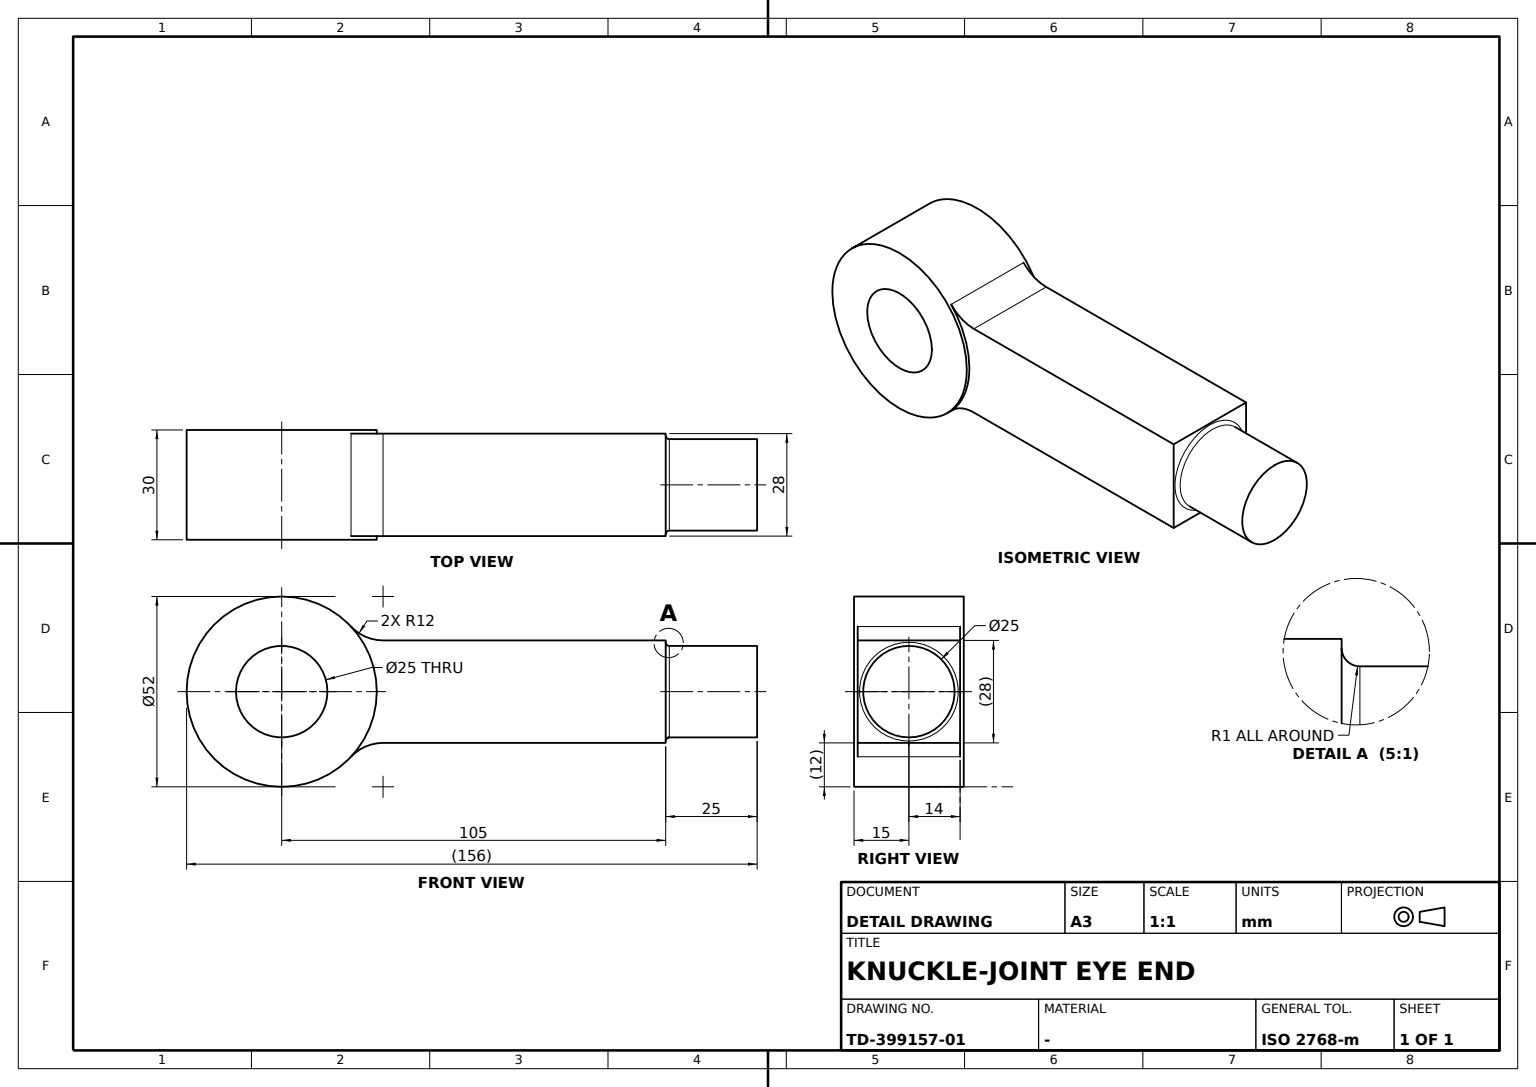
ISO-10303-21;
HEADER;
FILE_DESCRIPTION((''),'2;1');
FILE_NAME('','',(''),(''),'','','');
FILE_SCHEMA(('AUTOMOTIVE_DESIGN'));
ENDSEC;
DATA;
#1=APPLICATION_CONTEXT('');
#2=PRODUCT_CONTEXT('',#1,'mechanical');
#3=PRODUCT('','','',(#2));
#4=PRODUCT_DEFINITION_FORMATION('','',#3);
#5=PRODUCT_DEFINITION_CONTEXT('',#1,'design');
#6=PRODUCT_DEFINITION('','',#4,#5);
#7=PRODUCT_DEFINITION_SHAPE('','',#6);
#8=(LENGTH_UNIT()NAMED_UNIT(*)SI_UNIT(.MILLI.,.METRE.));
#9=(NAMED_UNIT(*)PLANE_ANGLE_UNIT()SI_UNIT($,.RADIAN.));
#10=(NAMED_UNIT(*)SI_UNIT($,.STERADIAN.)SOLID_ANGLE_UNIT());
#11=UNCERTAINTY_MEASURE_WITH_UNIT(LENGTH_MEASURE(1.E-05),#8,'distance_accuracy_value','');
#12=(GEOMETRIC_REPRESENTATION_CONTEXT(3)GLOBAL_UNCERTAINTY_ASSIGNED_CONTEXT((#11))GLOBAL_UNIT_ASSIGNED_CONTEXT((#8,#9,#10))REPRESENTATION_CONTEXT('',''));
#13=CARTESIAN_POINT('',(0.,-26.,-15.));
#14=VERTEX_POINT('',#13);
#15=CARTESIAN_POINT('',(0.,26.,-15.));
#16=VERTEX_POINT('',#15);
#17=CARTESIAN_POINT('',(0.,0.,-15.));
#18=DIRECTION('',(0.,0.,1.));
#19=DIRECTION('',(0.,-1.,0.));
#20=AXIS2_PLACEMENT_3D('',#17,#18,#19);
#21=CIRCLE('',#20,26.);
#22=EDGE_CURVE('',#14,#16,#21,.T.);
#23=ORIENTED_EDGE('',*,*,#22,.F.);
#24=EDGE_CURVE('',#16,#14,#21,.T.);
#25=ORIENTED_EDGE('',*,*,#24,.F.);
#26=EDGE_LOOP('',(#23,#25));
#27=FACE_OUTER_BOUND('',#26,.T.);
#28=CARTESIAN_POINT('',(0.,12.5,-15.));
#29=VERTEX_POINT('',#28);
#30=CARTESIAN_POINT('',(0.,-12.5,-15.));
#31=VERTEX_POINT('',#30);
#32=CIRCLE('',#20,12.5);
#33=EDGE_CURVE('',#29,#31,#32,.T.);
#34=ORIENTED_EDGE('',*,*,#33,.T.);
#35=EDGE_CURVE('',#31,#29,#32,.T.);
#36=ORIENTED_EDGE('',*,*,#35,.T.);
#37=EDGE_LOOP('',(#34,#36));
#38=FACE_BOUND('',#37,.T.);
#39=PLANE('',#20);
#40=ADVANCED_FACE('',(#27,#38),#39,.F.);
#41=CARTESIAN_POINT('',(0.,-12.5,14.));
#42=VERTEX_POINT('',#41);
#43=CARTESIAN_POINT('',(0.,-12.5,-14.));
#44=VERTEX_POINT('',#43);
#45=CARTESIAN_POINT('',(0.,-12.5,6.84));
#46=DIRECTION('',(0.,0.,-1.));
#47=VECTOR('',#46,1000.);
#48=LINE('',#45,#47);
#49=EDGE_CURVE('',#42,#44,#48,.T.);
#50=ORIENTED_EDGE('',*,*,#49,.F.);
#51=CARTESIAN_POINT('',(0.,12.5,14.));
#52=VERTEX_POINT('',#51);
#53=CARTESIAN_POINT('',(0.,0.,14.));
#54=DIRECTION('',(0.,1.,0.));
#55=AXIS2_PLACEMENT_3D('',#53,#18,#54);
#56=CIRCLE('',#55,12.5);
#57=EDGE_CURVE('',#42,#52,#56,.T.);
#58=ORIENTED_EDGE('',*,*,#57,.T.);
#59=CARTESIAN_POINT('',(0.,12.5,-14.));
#60=VERTEX_POINT('',#59);
#61=CARTESIAN_POINT('',(0.,12.5,6.84));
#62=LINE('',#61,#47);
#63=EDGE_CURVE('',#52,#60,#62,.T.);
#64=ORIENTED_EDGE('',*,*,#63,.T.);
#65=CARTESIAN_POINT('',(0.,0.,-14.));
#66=AXIS2_PLACEMENT_3D('',#65,#18,#54);
#67=CIRCLE('',#66,12.5);
#68=EDGE_CURVE('',#44,#60,#67,.T.);
#69=ORIENTED_EDGE('',*,*,#68,.F.);
#70=EDGE_LOOP('',(#50,#58,#64,#69));
#71=FACE_OUTER_BOUND('',#70,.T.);
#72=CARTESIAN_POINT('',(0.,0.,6.84));
#73=AXIS2_PLACEMENT_3D('',#72,#46,#54);
#74=CYLINDRICAL_SURFACE('',#73,12.5);
#75=ADVANCED_FACE('',(#71),#74,.F.);
#76=CARTESIAN_POINT('',(0.,12.5,15.));
#77=VERTEX_POINT('',#76);
#78=CARTESIAN_POINT('',(0.,-12.5,15.));
#79=VERTEX_POINT('',#78);
#80=CARTESIAN_POINT('',(0.,0.,15.));
#81=AXIS2_PLACEMENT_3D('',#80,#18,#19);
#82=CIRCLE('',#81,12.5);
#83=EDGE_CURVE('',#77,#79,#82,.T.);
#84=ORIENTED_EDGE('',*,*,#83,.F.);
#85=EDGE_CURVE('',#79,#77,#82,.T.);
#86=ORIENTED_EDGE('',*,*,#85,.F.);
#87=EDGE_LOOP('',(#84,#86));
#88=FACE_BOUND('',#87,.T.);
#89=CARTESIAN_POINT('',(0.,26.,15.));
#90=VERTEX_POINT('',#89);
#91=CARTESIAN_POINT('',(0.,-26.,15.));
#92=VERTEX_POINT('',#91);
#93=CIRCLE('',#81,26.);
#94=EDGE_CURVE('',#90,#92,#93,.T.);
#95=ORIENTED_EDGE('',*,*,#94,.T.);
#96=EDGE_CURVE('',#92,#90,#93,.T.);
#97=ORIENTED_EDGE('',*,*,#96,.T.);
#98=EDGE_LOOP('',(#95,#97));
#99=FACE_OUTER_BOUND('',#98,.T.);
#100=PLANE('',#81);
#101=ADVANCED_FACE('',(#88,#99),#100,.T.);
#102=ORIENTED_EDGE('',*,*,#63,.F.);
#103=EDGE_CURVE('',#52,#42,#56,.T.);
#104=ORIENTED_EDGE('',*,*,#103,.T.);
#105=ORIENTED_EDGE('',*,*,#49,.T.);
#106=EDGE_CURVE('',#60,#44,#67,.T.);
#107=ORIENTED_EDGE('',*,*,#106,.F.);
#108=EDGE_LOOP('',(#102,#104,#105,#107));
#109=FACE_OUTER_BOUND('',#108,.T.);
#110=ADVANCED_FACE('',(#109),#74,.F.);
#111=CARTESIAN_POINT('',(12.5,106.,0.));
#112=VERTEX_POINT('',#111);
#113=CARTESIAN_POINT('',(-12.5,106.,0.));
#114=VERTEX_POINT('',#113);
#115=CARTESIAN_POINT('',(0.,106.,0.));
#116=DIRECTION('',(-1.,0.,0.));
#117=AXIS2_PLACEMENT_3D('',#115,#19,#116);
#118=CIRCLE('',#117,12.5);
#119=EDGE_CURVE('',#112,#114,#118,.T.);
#120=ORIENTED_EDGE('',*,*,#119,.F.);
#121=CARTESIAN_POINT('',(12.5,130.,0.));
#122=VERTEX_POINT('',#121);
#123=CARTESIAN_POINT('',(12.5,117.5,0.));
#124=VECTOR('',#54,1000.);
#125=LINE('',#123,#124);
#126=EDGE_CURVE('',#112,#122,#125,.T.);
#127=ORIENTED_EDGE('',*,*,#126,.T.);
#128=CARTESIAN_POINT('',(-12.5,130.,0.));
#129=VERTEX_POINT('',#128);
#130=CARTESIAN_POINT('',(0.,130.,0.));
#131=AXIS2_PLACEMENT_3D('',#130,#54,#116);
#132=CIRCLE('',#131,12.5);
#133=EDGE_CURVE('',#129,#122,#132,.T.);
#134=ORIENTED_EDGE('',*,*,#133,.F.);
#135=CARTESIAN_POINT('',(-12.5,117.5,0.));
#136=LINE('',#135,#124);
#137=EDGE_CURVE('',#114,#129,#136,.T.);
#138=ORIENTED_EDGE('',*,*,#137,.F.);
#139=EDGE_LOOP('',(#120,#127,#134,#138));
#140=FACE_OUTER_BOUND('',#139,.T.);
#141=CARTESIAN_POINT('',(0.,117.5,0.));
#142=AXIS2_PLACEMENT_3D('',#141,#19,#116);
#143=CYLINDRICAL_SURFACE('',#142,12.5);
#144=ADVANCED_FACE('',(#140),#143,.T.);
#145=CARTESIAN_POINT('',(0.,-12.5,0.));
#146=VECTOR('',#18,1000.);
#147=LINE('',#145,#146);
#148=EDGE_CURVE('',#42,#79,#147,.T.);
#149=ORIENTED_EDGE('',*,*,#148,.F.);
#150=ORIENTED_EDGE('',*,*,#103,.F.);
#151=CARTESIAN_POINT('',(0.,12.5,0.));
#152=LINE('',#151,#146);
#153=EDGE_CURVE('',#52,#77,#152,.T.);
#154=ORIENTED_EDGE('',*,*,#153,.T.);
#155=ORIENTED_EDGE('',*,*,#83,.T.);
#156=EDGE_LOOP('',(#149,#150,#154,#155));
#157=FACE_OUTER_BOUND('',#156,.T.);
#158=CARTESIAN_POINT('',(0.,0.,0.));
#159=AXIS2_PLACEMENT_3D('',#158,#46,#19);
#160=CYLINDRICAL_SURFACE('',#159,12.5);
#161=ADVANCED_FACE('',(#157),#160,.F.);
#162=EDGE_CURVE('',#31,#44,#147,.T.);
#163=ORIENTED_EDGE('',*,*,#162,.F.);
#164=ORIENTED_EDGE('',*,*,#33,.F.);
#165=EDGE_CURVE('',#29,#60,#152,.T.);
#166=ORIENTED_EDGE('',*,*,#165,.T.);
#167=ORIENTED_EDGE('',*,*,#106,.T.);
#168=EDGE_LOOP('',(#163,#164,#166,#167));
#169=FACE_OUTER_BOUND('',#168,.T.);
#170=ADVANCED_FACE('',(#169),#160,.F.);
#171=ORIENTED_EDGE('',*,*,#137,.T.);
#172=EDGE_CURVE('',#122,#129,#132,.T.);
#173=ORIENTED_EDGE('',*,*,#172,.F.);
#174=ORIENTED_EDGE('',*,*,#126,.F.);
#175=EDGE_CURVE('',#114,#112,#118,.T.);
#176=ORIENTED_EDGE('',*,*,#175,.F.);
#177=EDGE_LOOP('',(#171,#173,#174,#176));
#178=FACE_OUTER_BOUND('',#177,.T.);
#179=ADVANCED_FACE('',(#178),#143,.T.);
#180=CARTESIAN_POINT('',(0.,26.,-14.));
#181=VERTEX_POINT('',#180);
#182=CARTESIAN_POINT('',(0.,26.,0.));
#183=LINE('',#182,#146);
#184=EDGE_CURVE('',#16,#181,#183,.T.);
#185=ORIENTED_EDGE('',*,*,#184,.F.);
#186=ORIENTED_EDGE('',*,*,#24,.T.);
#187=CARTESIAN_POINT('',(0.,-26.,0.));
#188=LINE('',#187,#146);
#189=EDGE_CURVE('',#14,#92,#188,.T.);
#190=ORIENTED_EDGE('',*,*,#189,.T.);
#191=ORIENTED_EDGE('',*,*,#94,.F.);
#192=CARTESIAN_POINT('',(0.,26.,14.));
#193=VERTEX_POINT('',#192);
#194=EDGE_CURVE('',#193,#90,#183,.T.);
#195=ORIENTED_EDGE('',*,*,#194,.F.);
#196=CARTESIAN_POINT('',(-17.789474,18.961398,14.));
#197=VERTEX_POINT('',#196);
#198=CIRCLE('',#55,26.);
#199=EDGE_CURVE('',#193,#197,#198,.T.);
#200=ORIENTED_EDGE('',*,*,#199,.T.);
#201=CARTESIAN_POINT('',(-17.789474,18.961398,-14.));
#202=VERTEX_POINT('',#201);
#203=CARTESIAN_POINT('',(-17.789474,18.961398,0.));
#204=LINE('',#203,#146);
#205=EDGE_CURVE('',#202,#197,#204,.T.);
#206=ORIENTED_EDGE('',*,*,#205,.F.);
#207=CIRCLE('',#66,26.);
#208=EDGE_CURVE('',#181,#202,#207,.T.);
#209=ORIENTED_EDGE('',*,*,#208,.F.);
#210=EDGE_LOOP('',(#185,#186,#190,#191,#195,#200,#206,#209));
#211=FACE_OUTER_BOUND('',#210,.T.);
#212=CYLINDRICAL_SURFACE('',#159,26.);
#213=ADVANCED_FACE('',(#211),#212,.T.);
#214=ORIENTED_EDGE('',*,*,#165,.F.);
#215=ORIENTED_EDGE('',*,*,#35,.F.);
#216=ORIENTED_EDGE('',*,*,#162,.T.);
#217=ORIENTED_EDGE('',*,*,#68,.T.);
#218=EDGE_LOOP('',(#214,#215,#216,#217));
#219=FACE_OUTER_BOUND('',#218,.T.);
#220=ADVANCED_FACE('',(#219),#160,.F.);
#221=ORIENTED_EDGE('',*,*,#199,.F.);
#222=CARTESIAN_POINT('',(17.789474,18.961398,14.));
#223=VERTEX_POINT('',#222);
#224=EDGE_CURVE('',#223,#193,#198,.T.);
#225=ORIENTED_EDGE('',*,*,#224,.F.);
#226=CARTESIAN_POINT('',(14.,27.712813,14.));
#227=VERTEX_POINT('',#226);
#228=CARTESIAN_POINT('',(26.,27.712813,14.));
#229=AXIS2_PLACEMENT_3D('',#228,#46,#54);
#230=CIRCLE('',#229,12.);
#231=EDGE_CURVE('',#223,#227,#230,.T.);
#232=ORIENTED_EDGE('',*,*,#231,.T.);
#233=CARTESIAN_POINT('',(14.,105.,14.));
#234=VERTEX_POINT('',#233);
#235=CARTESIAN_POINT('',(14.,66.356406,14.));
#236=LINE('',#235,#124);
#237=EDGE_CURVE('',#227,#234,#236,.T.);
#238=ORIENTED_EDGE('',*,*,#237,.T.);
#239=CARTESIAN_POINT('',(-14.,105.,14.));
#240=VERTEX_POINT('',#239);
#241=CARTESIAN_POINT('',(0.,105.,14.));
#242=VECTOR('',#116,1000.);
#243=LINE('',#241,#242);
#244=EDGE_CURVE('',#234,#240,#243,.T.);
#245=ORIENTED_EDGE('',*,*,#244,.T.);
#246=CARTESIAN_POINT('',(-14.,27.712813,14.));
#247=VERTEX_POINT('',#246);
#248=CARTESIAN_POINT('',(-14.,66.356406,14.));
#249=VECTOR('',#19,1000.);
#250=LINE('',#248,#249);
#251=EDGE_CURVE('',#240,#247,#250,.T.);
#252=ORIENTED_EDGE('',*,*,#251,.T.);
#253=CARTESIAN_POINT('',(-26.,27.712813,14.));
#254=AXIS2_PLACEMENT_3D('',#253,#46,#54);
#255=CIRCLE('',#254,12.);
#256=EDGE_CURVE('',#247,#197,#255,.T.);
#257=ORIENTED_EDGE('',*,*,#256,.T.);
#258=EDGE_LOOP('',(#221,#225,#232,#238,#245,#252,#257));
#259=FACE_OUTER_BOUND('',#258,.T.);
#260=PLANE('',#55);
#261=ADVANCED_FACE('',(#259),#260,.T.);
#262=CARTESIAN_POINT('',(13.5,105.,0.));
#263=VERTEX_POINT('',#262);
#264=CARTESIAN_POINT('',(-13.5,105.,0.));
#265=VERTEX_POINT('',#264);
#266=CARTESIAN_POINT('',(0.,105.,0.));
#267=DIRECTION('',(1.,0.,0.));
#268=AXIS2_PLACEMENT_3D('',#266,#19,#267);
#269=CIRCLE('',#268,13.5);
#270=EDGE_CURVE('',#263,#265,#269,.T.);
#271=ORIENTED_EDGE('',*,*,#270,.T.);
#272=EDGE_CURVE('',#265,#263,#269,.T.);
#273=ORIENTED_EDGE('',*,*,#272,.T.);
#274=EDGE_LOOP('',(#271,#273));
#275=FACE_BOUND('',#274,.T.);
#276=CARTESIAN_POINT('',(14.,105.,-14.));
#277=VERTEX_POINT('',#276);
#278=CARTESIAN_POINT('',(14.,105.,0.));
#279=LINE('',#278,#146);
#280=EDGE_CURVE('',#277,#234,#279,.T.);
#281=ORIENTED_EDGE('',*,*,#280,.F.);
#282=CARTESIAN_POINT('',(-14.,105.,-14.));
#283=VERTEX_POINT('',#282);
#284=CARTESIAN_POINT('',(0.,105.,-14.));
#285=LINE('',#284,#242);
#286=EDGE_CURVE('',#277,#283,#285,.T.);
#287=ORIENTED_EDGE('',*,*,#286,.T.);
#288=CARTESIAN_POINT('',(-14.,105.,0.));
#289=LINE('',#288,#146);
#290=EDGE_CURVE('',#283,#240,#289,.T.);
#291=ORIENTED_EDGE('',*,*,#290,.T.);
#292=ORIENTED_EDGE('',*,*,#244,.F.);
#293=EDGE_LOOP('',(#281,#287,#291,#292));
#294=FACE_OUTER_BOUND('',#293,.T.);
#295=AXIS2_PLACEMENT_3D('',#288,#19,#267);
#296=PLANE('',#295);
#297=ADVANCED_FACE('',(#275,#294),#296,.F.);
#298=ORIENTED_EDGE('',*,*,#237,.F.);
#299=CARTESIAN_POINT('',(14.,27.712813,-14.));
#300=VERTEX_POINT('',#299);
#301=CARTESIAN_POINT('',(14.,27.712813,0.));
#302=LINE('',#301,#146);
#303=EDGE_CURVE('',#300,#227,#302,.T.);
#304=ORIENTED_EDGE('',*,*,#303,.F.);
#305=CARTESIAN_POINT('',(14.,66.356406,-14.));
#306=LINE('',#305,#124);
#307=EDGE_CURVE('',#300,#277,#306,.T.);
#308=ORIENTED_EDGE('',*,*,#307,.T.);
#309=ORIENTED_EDGE('',*,*,#280,.T.);
#310=EDGE_LOOP('',(#298,#304,#308,#309));
#311=FACE_OUTER_BOUND('',#310,.T.);
#312=AXIS2_PLACEMENT_3D('',#278,#116,#19);
#313=PLANE('',#312);
#314=ADVANCED_FACE('',(#311),#313,.F.);
#315=CARTESIAN_POINT('',(17.789474,18.961398,-14.));
#316=VERTEX_POINT('',#315);
#317=CARTESIAN_POINT('',(17.789474,18.961398,0.));
#318=LINE('',#317,#146);
#319=EDGE_CURVE('',#316,#223,#318,.T.);
#320=ORIENTED_EDGE('',*,*,#319,.F.);
#321=CARTESIAN_POINT('',(26.,27.712813,-14.));
#322=AXIS2_PLACEMENT_3D('',#321,#46,#54);
#323=CIRCLE('',#322,12.);
#324=EDGE_CURVE('',#316,#300,#323,.T.);
#325=ORIENTED_EDGE('',*,*,#324,.T.);
#326=ORIENTED_EDGE('',*,*,#303,.T.);
#327=ORIENTED_EDGE('',*,*,#231,.F.);
#328=EDGE_LOOP('',(#320,#325,#326,#327));
#329=FACE_OUTER_BOUND('',#328,.T.);
#330=CARTESIAN_POINT('',(26.,27.712813,0.));
#331=AXIS2_PLACEMENT_3D('',#330,#46,#54);
#332=CYLINDRICAL_SURFACE('',#331,12.);
#333=ADVANCED_FACE('',(#329),#332,.F.);
#334=ORIENTED_EDGE('',*,*,#22,.T.);
#335=ORIENTED_EDGE('',*,*,#184,.T.);
#336=EDGE_CURVE('',#316,#181,#207,.T.);
#337=ORIENTED_EDGE('',*,*,#336,.F.);
#338=ORIENTED_EDGE('',*,*,#319,.T.);
#339=ORIENTED_EDGE('',*,*,#224,.T.);
#340=ORIENTED_EDGE('',*,*,#194,.T.);
#341=ORIENTED_EDGE('',*,*,#96,.F.);
#342=ORIENTED_EDGE('',*,*,#189,.F.);
#343=EDGE_LOOP('',(#334,#335,#337,#338,#339,#340,#341,#342));
#344=FACE_OUTER_BOUND('',#343,.T.);
#345=ADVANCED_FACE('',(#344),#212,.T.);
#346=ORIENTED_EDGE('',*,*,#119,.T.);
#347=CARTESIAN_POINT('',(-13.5,106.,0.));
#348=AXIS2_PLACEMENT_3D('',#347,#46,#116);
#349=CIRCLE('',#348,1.);
#350=EDGE_CURVE('',#114,#265,#349,.T.);
#351=ORIENTED_EDGE('',*,*,#350,.T.);
#352=ORIENTED_EDGE('',*,*,#270,.F.);
#353=CARTESIAN_POINT('',(13.5,106.,0.));
#354=DIRECTION('',(0.000000025,0.,1.));
#355=DIRECTION('',(1.,0.,-0.000000025));
#356=AXIS2_PLACEMENT_3D('',#353,#354,#355);
#357=CIRCLE('',#356,1.);
#358=EDGE_CURVE('',#112,#263,#357,.T.);
#359=ORIENTED_EDGE('',*,*,#358,.F.);
#360=EDGE_LOOP('',(#346,#351,#352,#359));
#361=FACE_OUTER_BOUND('',#360,.T.);
#362=DIRECTION('',(0.590104672,0.,-0.807326747));
#363=AXIS2_PLACEMENT_3D('',#115,#19,#362);
#364=TOROIDAL_SURFACE('',#363,13.5,1.);
#365=ADVANCED_FACE('',(#361),#364,.F.);
#366=CARTESIAN_POINT('',(-14.,27.712813,-14.));
#367=VERTEX_POINT('',#366);
#368=CARTESIAN_POINT('',(-14.,66.356406,-14.));
#369=LINE('',#368,#249);
#370=EDGE_CURVE('',#283,#367,#369,.T.);
#371=ORIENTED_EDGE('',*,*,#370,.T.);
#372=CARTESIAN_POINT('',(-14.,27.712813,0.));
#373=LINE('',#372,#146);
#374=EDGE_CURVE('',#367,#247,#373,.T.);
#375=ORIENTED_EDGE('',*,*,#374,.T.);
#376=ORIENTED_EDGE('',*,*,#251,.F.);
#377=ORIENTED_EDGE('',*,*,#290,.F.);
#378=EDGE_LOOP('',(#371,#375,#376,#377));
#379=FACE_OUTER_BOUND('',#378,.T.);
#380=AXIS2_PLACEMENT_3D('',#372,#267,#54);
#381=PLANE('',#380);
#382=ADVANCED_FACE('',(#379),#381,.F.);
#383=ORIENTED_EDGE('',*,*,#208,.T.);
#384=CARTESIAN_POINT('',(-26.,27.712813,-14.));
#385=AXIS2_PLACEMENT_3D('',#384,#46,#54);
#386=CIRCLE('',#385,12.);
#387=EDGE_CURVE('',#367,#202,#386,.T.);
#388=ORIENTED_EDGE('',*,*,#387,.F.);
#389=ORIENTED_EDGE('',*,*,#370,.F.);
#390=ORIENTED_EDGE('',*,*,#286,.F.);
#391=ORIENTED_EDGE('',*,*,#307,.F.);
#392=ORIENTED_EDGE('',*,*,#324,.F.);
#393=ORIENTED_EDGE('',*,*,#336,.T.);
#394=EDGE_LOOP('',(#383,#388,#389,#390,#391,#392,#393));
#395=FACE_OUTER_BOUND('',#394,.T.);
#396=PLANE('',#66);
#397=ADVANCED_FACE('',(#395),#396,.F.);
#398=ORIENTED_EDGE('',*,*,#57,.F.);
#399=ORIENTED_EDGE('',*,*,#148,.T.);
#400=ORIENTED_EDGE('',*,*,#85,.T.);
#401=ORIENTED_EDGE('',*,*,#153,.F.);
#402=EDGE_LOOP('',(#398,#399,#400,#401));
#403=FACE_OUTER_BOUND('',#402,.T.);
#404=ADVANCED_FACE('',(#403),#160,.F.);
#405=ORIENTED_EDGE('',*,*,#133,.T.);
#406=ORIENTED_EDGE('',*,*,#172,.T.);
#407=EDGE_LOOP('',(#405,#406));
#408=FACE_OUTER_BOUND('',#407,.T.);
#409=PLANE('',#131);
#410=ADVANCED_FACE('',(#408),#409,.T.);
#411=ORIENTED_EDGE('',*,*,#205,.T.);
#412=ORIENTED_EDGE('',*,*,#256,.F.);
#413=ORIENTED_EDGE('',*,*,#374,.F.);
#414=ORIENTED_EDGE('',*,*,#387,.T.);
#415=EDGE_LOOP('',(#411,#412,#413,#414));
#416=FACE_OUTER_BOUND('',#415,.T.);
#417=CARTESIAN_POINT('',(-26.,27.712813,0.));
#418=AXIS2_PLACEMENT_3D('',#417,#46,#54);
#419=CYLINDRICAL_SURFACE('',#418,12.);
#420=ADVANCED_FACE('',(#416),#419,.F.);
#421=ORIENTED_EDGE('',*,*,#272,.F.);
#422=ORIENTED_EDGE('',*,*,#350,.F.);
#423=ORIENTED_EDGE('',*,*,#175,.T.);
#424=ORIENTED_EDGE('',*,*,#358,.T.);
#425=EDGE_LOOP('',(#421,#422,#423,#424));
#426=FACE_OUTER_BOUND('',#425,.T.);
#427=DIRECTION('',(-0.661171515,0.,0.750234782));
#428=AXIS2_PLACEMENT_3D('',#115,#19,#427);
#429=TOROIDAL_SURFACE('',#428,13.5,1.);
#430=ADVANCED_FACE('',(#426),#429,.F.);
#431=CLOSED_SHELL('',(#40,#75,#101,#110,#144,#161,#170,#179,#213,#220,#261,#297,#314,#333,#345,#365,#382,#397,#404,#410,#420,#430));
#432=MANIFOLD_SOLID_BREP('',#431);
#433=ADVANCED_BREP_SHAPE_REPRESENTATION('',(#432),#12);
#434=SHAPE_DEFINITION_REPRESENTATION(#7,#433);
ENDSEC;
END-ISO-10303-21;
